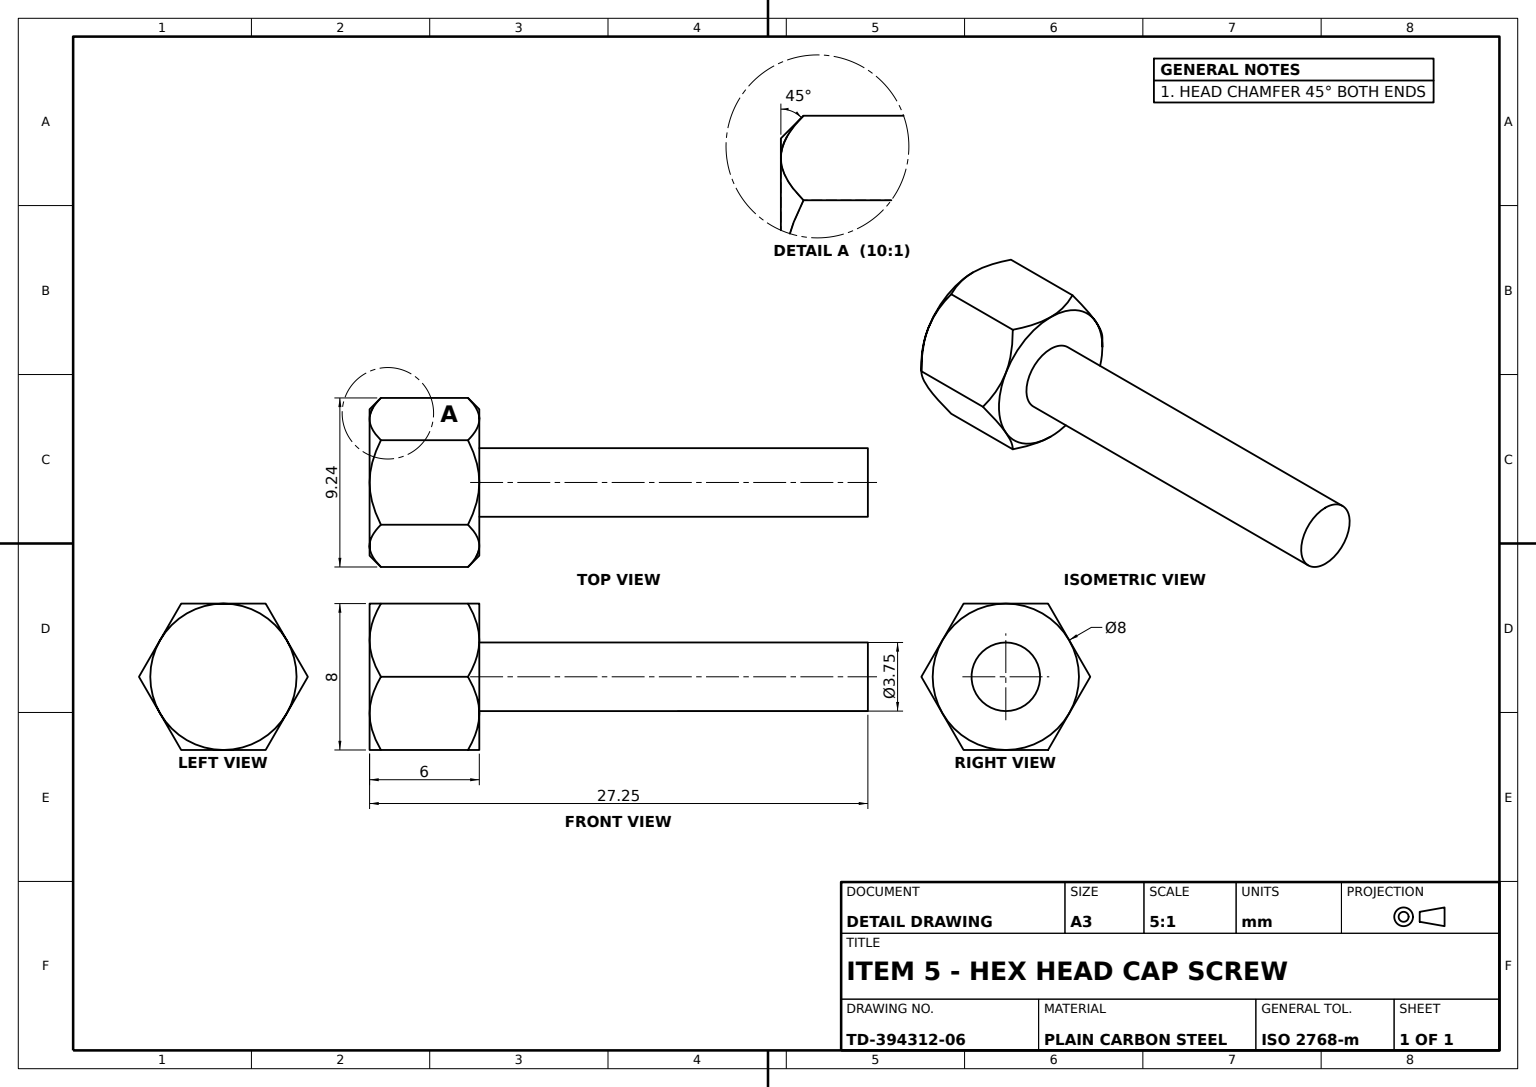
ISO-10303-21;
HEADER;
FILE_DESCRIPTION((''),'2;1');
FILE_NAME('','',(''),(''),'','','');
FILE_SCHEMA(('AUTOMOTIVE_DESIGN'));
ENDSEC;
DATA;
#1=APPLICATION_CONTEXT('');
#2=PRODUCT_CONTEXT('',#1,'mechanical');
#3=PRODUCT('','','',(#2));
#4=PRODUCT_DEFINITION_FORMATION('','',#3);
#5=PRODUCT_DEFINITION_CONTEXT('',#1,'design');
#6=PRODUCT_DEFINITION('','',#4,#5);
#7=PRODUCT_DEFINITION_SHAPE('','',#6);
#8=(LENGTH_UNIT()NAMED_UNIT(*)SI_UNIT(.MILLI.,.METRE.));
#9=(NAMED_UNIT(*)PLANE_ANGLE_UNIT()SI_UNIT($,.RADIAN.));
#10=(NAMED_UNIT(*)SI_UNIT($,.STERADIAN.)SOLID_ANGLE_UNIT());
#11=UNCERTAINTY_MEASURE_WITH_UNIT(LENGTH_MEASURE(1.E-05),#8,'distance_accuracy_value','');
#12=(GEOMETRIC_REPRESENTATION_CONTEXT(3)GLOBAL_UNCERTAINTY_ASSIGNED_CONTEXT((#11))GLOBAL_UNIT_ASSIGNED_CONTEXT((#8,#9,#10))REPRESENTATION_CONTEXT('',''));
#13=CARTESIAN_POINT('',(-2.309401,5.381198,4.));
#14=VERTEX_POINT('',#13);
#15=CARTESIAN_POINT('',(-2.309401,0.618802,4.));
#16=VERTEX_POINT('',#15);
#17=CARTESIAN_POINT('',(-2.309401,6.,4.));
#18=DIRECTION('',(0.,-1.,0.));
#19=VECTOR('',#18,1000.);
#20=LINE('',#17,#19);
#21=EDGE_CURVE('',#14,#16,#20,.T.);
#22=ORIENTED_EDGE('',*,*,#21,.F.);
#23=CARTESIAN_POINT('',(-3.464102,6.,2.));
#24=VERTEX_POINT('',#23);
#25=CARTESIAN_POINT('',(-3.263253,6.,2.34788));
#26=CARTESIAN_POINT('',(-3.065819,5.938579,2.689845));
#27=CARTESIAN_POINT('',(-2.67643,5.717205,3.364287));
#28=CARTESIAN_POINT('',(-2.490265,5.562062,3.686735));
#29=B_SPLINE_CURVE_WITH_KNOTS('',3,(#23,#25,#26,#27,#28,#13),.UNSPECIFIED.,.F.,.F.,(4,2,4),(0.002394158,0.003582724,0.00477129),.UNSPECIFIED.);
#30=EDGE_CURVE('',#24,#14,#29,.T.);
#31=ORIENTED_EDGE('',*,*,#30,.F.);
#32=CARTESIAN_POINT('',(-4.618802,5.381198,0.));
#33=VERTEX_POINT('',#32);
#34=CARTESIAN_POINT('',(-4.437729,5.562271,0.313628));
#35=CARTESIAN_POINT('',(-4.252558,5.716136,0.634354));
#36=CARTESIAN_POINT('',(-3.964816,5.880647,1.132738));
#37=CARTESIAN_POINT('',(-3.86722,5.924319,1.301778));
#38=CARTESIAN_POINT('',(-3.667881,5.984124,1.647044));
#39=CARTESIAN_POINT('',(-3.565234,6.,1.824833));
#40=B_SPLINE_CURVE_WITH_KNOTS('',3,(#32,#34,#35,#36,#37,#38,#39,#23),.UNSPECIFIED.,.F.,.F.,(4,2,2,4),(0.000000254,0.001197206,0.001795682,0.002394158),.UNSPECIFIED.);
#41=EDGE_CURVE('',#33,#24,#40,.T.);
#42=ORIENTED_EDGE('',*,*,#41,.F.);
#43=CARTESIAN_POINT('',(-4.618802,0.618802,0.));
#44=VERTEX_POINT('',#43);
#45=CARTESIAN_POINT('',(-4.618802,6.,0.));
#46=LINE('',#45,#19);
#47=EDGE_CURVE('',#33,#44,#46,.T.);
#48=ORIENTED_EDGE('',*,*,#47,.T.);
#49=CARTESIAN_POINT('',(-3.464102,0.,2.));
#50=VERTEX_POINT('',#49);
#51=CARTESIAN_POINT('',(-3.66495,0.,1.65212));
#52=CARTESIAN_POINT('',(-3.862384,0.061421,1.310155));
#53=CARTESIAN_POINT('',(-4.251773,0.282795,0.635713));
#54=CARTESIAN_POINT('',(-4.437938,0.437938,0.313265));
#55=B_SPLINE_CURVE_WITH_KNOTS('',3,(#49,#51,#52,#53,#54,#43),.UNSPECIFIED.,.F.,.F.,(4,2,4),(0.002394158,0.003582724,0.00477129),.UNSPECIFIED.);
#56=EDGE_CURVE('',#50,#44,#55,.T.);
#57=ORIENTED_EDGE('',*,*,#56,.F.);
#58=CARTESIAN_POINT('',(-2.490474,0.437729,3.686372));
#59=CARTESIAN_POINT('',(-2.675646,0.283864,3.365646));
#60=CARTESIAN_POINT('',(-2.963387,0.119353,2.867262));
#61=CARTESIAN_POINT('',(-3.060983,0.075681,2.698222));
#62=CARTESIAN_POINT('',(-3.260323,0.015876,2.352956));
#63=CARTESIAN_POINT('',(-3.362969,0.,2.175167));
#64=B_SPLINE_CURVE_WITH_KNOTS('',3,(#15,#58,#59,#60,#61,#62,#63,#49),.UNSPECIFIED.,.F.,.F.,(4,2,2,4),(0.000000254,0.001197206,0.001795682,0.002394158),.UNSPECIFIED.);
#65=EDGE_CURVE('',#16,#50,#64,.T.);
#66=ORIENTED_EDGE('',*,*,#65,.F.);
#67=EDGE_LOOP('',(#22,#31,#42,#48,#57,#66));
#68=FACE_OUTER_BOUND('',#67,.T.);
#69=DIRECTION('',(0.866025404,0.,-0.5));
#70=DIRECTION('',(-0.5,0.,-0.866025404));
#71=AXIS2_PLACEMENT_3D('',#45,#69,#70);
#72=PLANE('',#71);
#73=ADVANCED_FACE('',(#68),#72,.F.);
#74=CARTESIAN_POINT('',(2.309401,5.381198,4.));
#75=VERTEX_POINT('',#74);
#76=CARTESIAN_POINT('',(3.464102,6.,2.));
#77=VERTEX_POINT('',#76);
#78=CARTESIAN_POINT('',(2.490474,5.562271,3.686372));
#79=CARTESIAN_POINT('',(2.675646,5.716136,3.365646));
#80=CARTESIAN_POINT('',(2.963387,5.880647,2.867262));
#81=CARTESIAN_POINT('',(3.060983,5.924319,2.698222));
#82=CARTESIAN_POINT('',(3.260323,5.984124,2.352956));
#83=CARTESIAN_POINT('',(3.362969,6.,2.175167));
#84=B_SPLINE_CURVE_WITH_KNOTS('',3,(#74,#78,#79,#80,#81,#82,#83,#76),.UNSPECIFIED.,.F.,.F.,(4,2,2,4),(0.000000254,0.001197206,0.001795682,0.002394158),.UNSPECIFIED.);
#85=EDGE_CURVE('',#75,#77,#84,.T.);
#86=ORIENTED_EDGE('',*,*,#85,.T.);
#87=CARTESIAN_POINT('',(0.,6.,4.));
#88=VERTEX_POINT('',#87);
#89=CARTESIAN_POINT('',(0.,6.,0.));
#90=DIRECTION('',(0.,1.,0.));
#91=DIRECTION('',(0.,0.,1.));
#92=AXIS2_PLACEMENT_3D('',#89,#90,#91);
#93=CIRCLE('',#92,4.);
#94=EDGE_CURVE('',#88,#77,#93,.T.);
#95=ORIENTED_EDGE('',*,*,#94,.F.);
#96=CARTESIAN_POINT('',(0.406277,6.,4.));
#97=CARTESIAN_POINT('',(0.803107,5.937088,4.));
#98=CARTESIAN_POINT('',(1.383908,5.771434,4.));
#99=CARTESIAN_POINT('',(1.576064,5.704089,4.));
#100=CARTESIAN_POINT('',(1.949047,5.553691,4.));
#101=CARTESIAN_POINT('',(2.130932,5.470433,4.));
#102=B_SPLINE_CURVE_WITH_KNOTS('',3,(#87,#96,#97,#98,#99,#100,#101,#74),.UNSPECIFIED.,.F.,.F.,(4,2,2,4),(0.012126845,0.013335171,0.013939334,0.014543496),.UNSPECIFIED.);
#103=EDGE_CURVE('',#88,#75,#102,.T.);
#104=ORIENTED_EDGE('',*,*,#103,.T.);
#105=EDGE_LOOP('',(#86,#95,#104));
#106=FACE_OUTER_BOUND('',#105,.T.);
#107=AXIS2_PLACEMENT_3D('',#89,#18,#91);
#108=CONICAL_SURFACE('',#107,4.,0.785398163);
#109=ADVANCED_FACE('',(#106),#108,.T.);
#110=CARTESIAN_POINT('',(0.,-21.25,-1.875));
#111=VERTEX_POINT('',#110);
#112=CARTESIAN_POINT('',(0.,0.,-1.875));
#113=VERTEX_POINT('',#112);
#114=VECTOR('',#90,1000.);
#115=LINE('',#110,#114);
#116=EDGE_CURVE('',#111,#113,#115,.T.);
#117=ORIENTED_EDGE('',*,*,#116,.F.);
#118=CARTESIAN_POINT('',(0.,-21.25,1.875));
#119=VERTEX_POINT('',#118);
#120=CARTESIAN_POINT('',(0.,-21.25,0.));
#121=DIRECTION('',(0.,0.,-1.));
#122=AXIS2_PLACEMENT_3D('',#120,#18,#121);
#123=CIRCLE('',#122,1.875);
#124=EDGE_CURVE('',#119,#111,#123,.T.);
#125=ORIENTED_EDGE('',*,*,#124,.F.);
#126=CARTESIAN_POINT('',(0.,0.,1.875));
#127=VERTEX_POINT('',#126);
#128=LINE('',#118,#114);
#129=EDGE_CURVE('',#119,#127,#128,.T.);
#130=ORIENTED_EDGE('',*,*,#129,.T.);
#131=CARTESIAN_POINT('',(0.,0.,0.));
#132=AXIS2_PLACEMENT_3D('',#131,#18,#121);
#133=CIRCLE('',#132,1.875);
#134=EDGE_CURVE('',#127,#113,#133,.T.);
#135=ORIENTED_EDGE('',*,*,#134,.T.);
#136=EDGE_LOOP('',(#117,#125,#130,#135));
#137=FACE_OUTER_BOUND('',#136,.T.);
#138=AXIS2_PLACEMENT_3D('',#120,#90,#91);
#139=CYLINDRICAL_SURFACE('',#138,1.875);
#140=ADVANCED_FACE('',(#137),#139,.T.);
#141=CARTESIAN_POINT('',(2.309401,5.381198,-4.));
#142=VERTEX_POINT('',#141);
#143=CARTESIAN_POINT('',(2.309401,0.618802,-4.));
#144=VERTEX_POINT('',#143);
#145=CARTESIAN_POINT('',(2.309401,6.,-4.));
#146=LINE('',#145,#19);
#147=EDGE_CURVE('',#142,#144,#146,.T.);
#148=ORIENTED_EDGE('',*,*,#147,.T.);
#149=CARTESIAN_POINT('',(0.,0.,-4.));
#150=VERTEX_POINT('',#149);
#151=CARTESIAN_POINT('',(0.406277,0.,-4.));
#152=CARTESIAN_POINT('',(0.803107,0.062912,-4.));
#153=CARTESIAN_POINT('',(1.383908,0.228566,-4.));
#154=CARTESIAN_POINT('',(1.576064,0.295911,-4.));
#155=CARTESIAN_POINT('',(1.949047,0.446309,-4.));
#156=CARTESIAN_POINT('',(2.130932,0.529567,-4.));
#157=B_SPLINE_CURVE_WITH_KNOTS('',3,(#149,#151,#152,#153,#154,#155,#156,#143),.UNSPECIFIED.,.F.,.F.,(4,2,2,4),(0.012126845,0.013335171,0.013939334,0.014543496),.UNSPECIFIED.);
#158=EDGE_CURVE('',#150,#144,#157,.T.);
#159=ORIENTED_EDGE('',*,*,#158,.F.);
#160=CARTESIAN_POINT('',(-2.309401,0.618802,-4.));
#161=VERTEX_POINT('',#160);
#162=CARTESIAN_POINT('',(-2.12979,0.528996,-4.));
#163=CARTESIAN_POINT('',(-1.94713,0.445459,-4.));
#164=CARTESIAN_POINT('',(-1.57371,0.295039,-4.));
#165=CARTESIAN_POINT('',(-1.381886,0.227903,-4.));
#166=CARTESIAN_POINT('',(-0.801056,0.062501,-4.));
#167=CARTESIAN_POINT('',(-0.405791,0.,-4.));
#168=B_SPLINE_CURVE_WITH_KNOTS('',3,(#160,#162,#163,#164,#165,#166,#167,#149),.UNSPECIFIED.,.F.,.F.,(4,2,2,4),(0.009713081,0.010316522,0.010919963,0.012126845),.UNSPECIFIED.);
#169=EDGE_CURVE('',#161,#150,#168,.T.);
#170=ORIENTED_EDGE('',*,*,#169,.F.);
#171=CARTESIAN_POINT('',(-2.309401,5.381198,-4.));
#172=VERTEX_POINT('',#171);
#173=CARTESIAN_POINT('',(-2.309401,6.,-4.));
#174=LINE('',#173,#19);
#175=EDGE_CURVE('',#172,#161,#174,.T.);
#176=ORIENTED_EDGE('',*,*,#175,.F.);
#177=CARTESIAN_POINT('',(0.,6.,-4.));
#178=VERTEX_POINT('',#177);
#179=CARTESIAN_POINT('',(-0.406277,6.,-4.));
#180=CARTESIAN_POINT('',(-0.803107,5.937088,-4.));
#181=CARTESIAN_POINT('',(-1.383908,5.771434,-4.));
#182=CARTESIAN_POINT('',(-1.576064,5.704089,-4.));
#183=CARTESIAN_POINT('',(-1.949047,5.553691,-4.));
#184=CARTESIAN_POINT('',(-2.130932,5.470433,-4.));
#185=B_SPLINE_CURVE_WITH_KNOTS('',3,(#177,#179,#180,#181,#182,#183,#184,#171),.UNSPECIFIED.,.F.,.F.,(4,2,2,4),(0.012126845,0.013335171,0.013939334,0.014543496),.UNSPECIFIED.);
#186=EDGE_CURVE('',#178,#172,#185,.T.);
#187=ORIENTED_EDGE('',*,*,#186,.F.);
#188=CARTESIAN_POINT('',(2.12979,5.471004,-4.));
#189=CARTESIAN_POINT('',(1.94713,5.554541,-4.));
#190=CARTESIAN_POINT('',(1.57371,5.704961,-4.));
#191=CARTESIAN_POINT('',(1.381886,5.772097,-4.));
#192=CARTESIAN_POINT('',(0.801056,5.937499,-4.));
#193=CARTESIAN_POINT('',(0.405791,6.,-4.));
#194=B_SPLINE_CURVE_WITH_KNOTS('',3,(#141,#188,#189,#190,#191,#192,#193,#177),.UNSPECIFIED.,.F.,.F.,(4,2,2,4),(0.009713081,0.010316522,0.010919963,0.012126845),.UNSPECIFIED.);
#195=EDGE_CURVE('',#142,#178,#194,.T.);
#196=ORIENTED_EDGE('',*,*,#195,.F.);
#197=EDGE_LOOP('',(#148,#159,#170,#176,#187,#196));
#198=FACE_OUTER_BOUND('',#197,.T.);
#199=DIRECTION('',(1.,0.,0.));
#200=AXIS2_PLACEMENT_3D('',#145,#91,#199);
#201=PLANE('',#200);
#202=ADVANCED_FACE('',(#198),#201,.F.);
#203=CARTESIAN_POINT('',(2.309401,0.618802,4.));
#204=VERTEX_POINT('',#203);
#205=CARTESIAN_POINT('',(2.309401,6.,4.));
#206=LINE('',#205,#19);
#207=EDGE_CURVE('',#75,#204,#206,.T.);
#208=ORIENTED_EDGE('',*,*,#207,.F.);
#209=ORIENTED_EDGE('',*,*,#103,.F.);
#210=CARTESIAN_POINT('',(-2.12979,5.471004,4.));
#211=CARTESIAN_POINT('',(-1.94713,5.554541,4.));
#212=CARTESIAN_POINT('',(-1.57371,5.704961,4.));
#213=CARTESIAN_POINT('',(-1.381886,5.772097,4.));
#214=CARTESIAN_POINT('',(-0.801056,5.937499,4.));
#215=CARTESIAN_POINT('',(-0.405791,6.,4.));
#216=B_SPLINE_CURVE_WITH_KNOTS('',3,(#13,#210,#211,#212,#213,#214,#215,#87),.UNSPECIFIED.,.F.,.F.,(4,2,2,4),(0.009713081,0.010316522,0.010919963,0.012126845),.UNSPECIFIED.);
#217=EDGE_CURVE('',#14,#88,#216,.T.);
#218=ORIENTED_EDGE('',*,*,#217,.F.);
#219=ORIENTED_EDGE('',*,*,#21,.T.);
#220=CARTESIAN_POINT('',(0.,0.,4.));
#221=VERTEX_POINT('',#220);
#222=CARTESIAN_POINT('',(-0.406277,0.,4.));
#223=CARTESIAN_POINT('',(-0.803107,0.062912,4.));
#224=CARTESIAN_POINT('',(-1.383908,0.228566,4.));
#225=CARTESIAN_POINT('',(-1.576064,0.295911,4.));
#226=CARTESIAN_POINT('',(-1.949047,0.446309,4.));
#227=CARTESIAN_POINT('',(-2.130932,0.529567,4.));
#228=B_SPLINE_CURVE_WITH_KNOTS('',3,(#220,#222,#223,#224,#225,#226,#227,#15),.UNSPECIFIED.,.F.,.F.,(4,2,2,4),(0.012126845,0.013335171,0.013939334,0.014543496),.UNSPECIFIED.);
#229=EDGE_CURVE('',#221,#16,#228,.T.);
#230=ORIENTED_EDGE('',*,*,#229,.F.);
#231=CARTESIAN_POINT('',(2.12979,0.528996,4.));
#232=CARTESIAN_POINT('',(1.94713,0.445459,4.));
#233=CARTESIAN_POINT('',(1.57371,0.295039,4.));
#234=CARTESIAN_POINT('',(1.381886,0.227903,4.));
#235=CARTESIAN_POINT('',(0.801056,0.062501,4.));
#236=CARTESIAN_POINT('',(0.405791,0.,4.));
#237=B_SPLINE_CURVE_WITH_KNOTS('',3,(#203,#231,#232,#233,#234,#235,#236,#220),.UNSPECIFIED.,.F.,.F.,(4,2,2,4),(0.009713081,0.010316522,0.010919963,0.012126845),.UNSPECIFIED.);
#238=EDGE_CURVE('',#204,#221,#237,.T.);
#239=ORIENTED_EDGE('',*,*,#238,.F.);
#240=EDGE_LOOP('',(#208,#209,#218,#219,#230,#239));
#241=FACE_OUTER_BOUND('',#240,.T.);
#242=DIRECTION('',(-1.,0.,0.));
#243=AXIS2_PLACEMENT_3D('',#17,#121,#242);
#244=PLANE('',#243);
#245=ADVANCED_FACE('',(#241),#244,.F.);
#246=CARTESIAN_POINT('',(-3.464102,0.,-2.));
#247=VERTEX_POINT('',#246);
#248=CARTESIAN_POINT('',(-4.437729,0.437729,-0.313628));
#249=CARTESIAN_POINT('',(-4.252558,0.283864,-0.634354));
#250=CARTESIAN_POINT('',(-3.964816,0.119353,-1.132738));
#251=CARTESIAN_POINT('',(-3.86722,0.075681,-1.301778));
#252=CARTESIAN_POINT('',(-3.667881,0.015876,-1.647044));
#253=CARTESIAN_POINT('',(-3.565234,0.,-1.824833));
#254=B_SPLINE_CURVE_WITH_KNOTS('',3,(#43,#248,#249,#250,#251,#252,#253,#246),.UNSPECIFIED.,.F.,.F.,(4,2,2,4),(0.000000254,0.001197206,0.001795682,0.002394158),.UNSPECIFIED.);
#255=EDGE_CURVE('',#44,#247,#254,.T.);
#256=ORIENTED_EDGE('',*,*,#255,.T.);
#257=AXIS2_PLACEMENT_3D('',#131,#90,#91);
#258=CIRCLE('',#257,4.);
#259=EDGE_CURVE('',#247,#50,#258,.T.);
#260=ORIENTED_EDGE('',*,*,#259,.T.);
#261=ORIENTED_EDGE('',*,*,#56,.T.);
#262=EDGE_LOOP('',(#256,#260,#261));
#263=FACE_OUTER_BOUND('',#262,.T.);
#264=AXIS2_PLACEMENT_3D('',#131,#90,#121);
#265=CONICAL_SURFACE('',#264,4.,0.785398163);
#266=ADVANCED_FACE('',(#263),#265,.T.);
#267=EDGE_CURVE('',#111,#119,#123,.T.);
#268=ORIENTED_EDGE('',*,*,#267,.F.);
#269=ORIENTED_EDGE('',*,*,#116,.T.);
#270=EDGE_CURVE('',#113,#127,#133,.T.);
#271=ORIENTED_EDGE('',*,*,#270,.T.);
#272=ORIENTED_EDGE('',*,*,#129,.F.);
#273=EDGE_LOOP('',(#268,#269,#271,#272));
#274=FACE_OUTER_BOUND('',#273,.T.);
#275=ADVANCED_FACE('',(#274),#139,.T.);
#276=CARTESIAN_POINT('',(3.464102,0.,-2.));
#277=VERTEX_POINT('',#276);
#278=CARTESIAN_POINT('',(4.618802,0.618802,0.));
#279=VERTEX_POINT('',#278);
#280=CARTESIAN_POINT('',(3.66495,0.,-1.65212));
#281=CARTESIAN_POINT('',(3.862384,0.061421,-1.310155));
#282=CARTESIAN_POINT('',(4.251773,0.282795,-0.635713));
#283=CARTESIAN_POINT('',(4.437938,0.437938,-0.313265));
#284=B_SPLINE_CURVE_WITH_KNOTS('',3,(#276,#280,#281,#282,#283,#278),.UNSPECIFIED.,.F.,.F.,(4,2,4),(0.002394158,0.003582724,0.00477129),.UNSPECIFIED.);
#285=EDGE_CURVE('',#277,#279,#284,.T.);
#286=ORIENTED_EDGE('',*,*,#285,.T.);
#287=CARTESIAN_POINT('',(3.464102,0.,2.));
#288=VERTEX_POINT('',#287);
#289=CARTESIAN_POINT('',(4.437729,0.437729,0.313628));
#290=CARTESIAN_POINT('',(4.252558,0.283864,0.634354));
#291=CARTESIAN_POINT('',(3.964816,0.119353,1.132738));
#292=CARTESIAN_POINT('',(3.86722,0.075681,1.301778));
#293=CARTESIAN_POINT('',(3.667881,0.015876,1.647044));
#294=CARTESIAN_POINT('',(3.565234,0.,1.824833));
#295=B_SPLINE_CURVE_WITH_KNOTS('',3,(#278,#289,#290,#291,#292,#293,#294,#287),.UNSPECIFIED.,.F.,.F.,(4,2,2,4),(0.000000254,0.001197206,0.001795682,0.002394158),.UNSPECIFIED.);
#296=EDGE_CURVE('',#279,#288,#295,.T.);
#297=ORIENTED_EDGE('',*,*,#296,.T.);
#298=EDGE_CURVE('',#288,#277,#258,.T.);
#299=ORIENTED_EDGE('',*,*,#298,.T.);
#300=EDGE_LOOP('',(#286,#297,#299));
#301=FACE_OUTER_BOUND('',#300,.T.);
#302=ADVANCED_FACE('',(#301),#265,.T.);
#303=CARTESIAN_POINT('',(-3.263253,0.,-2.34788));
#304=CARTESIAN_POINT('',(-3.065819,0.061421,-2.689845));
#305=CARTESIAN_POINT('',(-2.67643,0.282795,-3.364287));
#306=CARTESIAN_POINT('',(-2.490265,0.437938,-3.686735));
#307=B_SPLINE_CURVE_WITH_KNOTS('',3,(#246,#303,#304,#305,#306,#160),.UNSPECIFIED.,.F.,.F.,(4,2,4),(0.002394158,0.003582724,0.00477129),.UNSPECIFIED.);
#308=EDGE_CURVE('',#247,#161,#307,.T.);
#309=ORIENTED_EDGE('',*,*,#308,.F.);
#310=ORIENTED_EDGE('',*,*,#255,.F.);
#311=ORIENTED_EDGE('',*,*,#47,.F.);
#312=CARTESIAN_POINT('',(-3.464102,6.,-2.));
#313=VERTEX_POINT('',#312);
#314=CARTESIAN_POINT('',(-3.66495,6.,-1.65212));
#315=CARTESIAN_POINT('',(-3.862384,5.938579,-1.310155));
#316=CARTESIAN_POINT('',(-4.251773,5.717205,-0.635713));
#317=CARTESIAN_POINT('',(-4.437938,5.562062,-0.313265));
#318=B_SPLINE_CURVE_WITH_KNOTS('',3,(#312,#314,#315,#316,#317,#32),.UNSPECIFIED.,.F.,.F.,(4,2,4),(0.002394158,0.003582724,0.00477129),.UNSPECIFIED.);
#319=EDGE_CURVE('',#313,#33,#318,.T.);
#320=ORIENTED_EDGE('',*,*,#319,.F.);
#321=CARTESIAN_POINT('',(-2.490474,5.562271,-3.686372));
#322=CARTESIAN_POINT('',(-2.675646,5.716136,-3.365646));
#323=CARTESIAN_POINT('',(-2.963387,5.880647,-2.867262));
#324=CARTESIAN_POINT('',(-3.060983,5.924319,-2.698222));
#325=CARTESIAN_POINT('',(-3.260323,5.984124,-2.352956));
#326=CARTESIAN_POINT('',(-3.362969,6.,-2.175167));
#327=B_SPLINE_CURVE_WITH_KNOTS('',3,(#171,#321,#322,#323,#324,#325,#326,#312),.UNSPECIFIED.,.F.,.F.,(4,2,2,4),(0.000000254,0.001197206,0.001795682,0.002394158),.UNSPECIFIED.);
#328=EDGE_CURVE('',#172,#313,#327,.T.);
#329=ORIENTED_EDGE('',*,*,#328,.F.);
#330=ORIENTED_EDGE('',*,*,#175,.T.);
#331=EDGE_LOOP('',(#309,#310,#311,#320,#329,#330));
#332=FACE_OUTER_BOUND('',#331,.T.);
#333=DIRECTION('',(0.866025404,0.,0.5));
#334=DIRECTION('',(0.5,0.,-0.866025404));
#335=AXIS2_PLACEMENT_3D('',#173,#333,#334);
#336=PLANE('',#335);
#337=ADVANCED_FACE('',(#332),#336,.F.);
#338=ORIENTED_EDGE('',*,*,#147,.F.);
#339=CARTESIAN_POINT('',(3.464102,6.,-2.));
#340=VERTEX_POINT('',#339);
#341=CARTESIAN_POINT('',(3.263253,6.,-2.34788));
#342=CARTESIAN_POINT('',(3.065819,5.938579,-2.689845));
#343=CARTESIAN_POINT('',(2.67643,5.717205,-3.364287));
#344=CARTESIAN_POINT('',(2.490265,5.562062,-3.686735));
#345=B_SPLINE_CURVE_WITH_KNOTS('',3,(#339,#341,#342,#343,#344,#141),.UNSPECIFIED.,.F.,.F.,(4,2,4),(0.002394158,0.003582724,0.00477129),.UNSPECIFIED.);
#346=EDGE_CURVE('',#340,#142,#345,.T.);
#347=ORIENTED_EDGE('',*,*,#346,.F.);
#348=CARTESIAN_POINT('',(4.618802,5.381198,0.));
#349=VERTEX_POINT('',#348);
#350=CARTESIAN_POINT('',(4.437729,5.562271,-0.313628));
#351=CARTESIAN_POINT('',(4.252558,5.716136,-0.634354));
#352=CARTESIAN_POINT('',(3.964816,5.880647,-1.132738));
#353=CARTESIAN_POINT('',(3.86722,5.924319,-1.301778));
#354=CARTESIAN_POINT('',(3.667881,5.984124,-1.647044));
#355=CARTESIAN_POINT('',(3.565234,6.,-1.824833));
#356=B_SPLINE_CURVE_WITH_KNOTS('',3,(#348,#350,#351,#352,#353,#354,#355,#339),.UNSPECIFIED.,.F.,.F.,(4,2,2,4),(0.000000254,0.001197206,0.001795682,0.002394158),.UNSPECIFIED.);
#357=EDGE_CURVE('',#349,#340,#356,.T.);
#358=ORIENTED_EDGE('',*,*,#357,.F.);
#359=CARTESIAN_POINT('',(4.618802,6.,0.));
#360=LINE('',#359,#19);
#361=EDGE_CURVE('',#349,#279,#360,.T.);
#362=ORIENTED_EDGE('',*,*,#361,.T.);
#363=ORIENTED_EDGE('',*,*,#285,.F.);
#364=CARTESIAN_POINT('',(2.490474,0.437729,-3.686372));
#365=CARTESIAN_POINT('',(2.675646,0.283864,-3.365646));
#366=CARTESIAN_POINT('',(2.963387,0.119353,-2.867262));
#367=CARTESIAN_POINT('',(3.060983,0.075681,-2.698222));
#368=CARTESIAN_POINT('',(3.260323,0.015876,-2.352956));
#369=CARTESIAN_POINT('',(3.362969,0.,-2.175167));
#370=B_SPLINE_CURVE_WITH_KNOTS('',3,(#143,#364,#365,#366,#367,#368,#369,#276),.UNSPECIFIED.,.F.,.F.,(4,2,2,4),(0.000000254,0.001197206,0.001795682,0.002394158),.UNSPECIFIED.);
#371=EDGE_CURVE('',#144,#277,#370,.T.);
#372=ORIENTED_EDGE('',*,*,#371,.F.);
#373=EDGE_LOOP('',(#338,#347,#358,#362,#363,#372));
#374=FACE_OUTER_BOUND('',#373,.T.);
#375=DIRECTION('',(-0.866025404,0.,0.5));
#376=DIRECTION('',(0.5,0.,0.866025404));
#377=AXIS2_PLACEMENT_3D('',#359,#375,#376);
#378=PLANE('',#377);
#379=ADVANCED_FACE('',(#374),#378,.F.);
#380=ORIENTED_EDGE('',*,*,#217,.T.);
#381=EDGE_CURVE('',#24,#88,#93,.T.);
#382=ORIENTED_EDGE('',*,*,#381,.F.);
#383=ORIENTED_EDGE('',*,*,#30,.T.);
#384=EDGE_LOOP('',(#380,#382,#383));
#385=FACE_OUTER_BOUND('',#384,.T.);
#386=ADVANCED_FACE('',(#385),#108,.T.);
#387=ORIENTED_EDGE('',*,*,#371,.T.);
#388=CIRCLE('',#132,4.);
#389=EDGE_CURVE('',#150,#277,#388,.T.);
#390=ORIENTED_EDGE('',*,*,#389,.F.);
#391=ORIENTED_EDGE('',*,*,#158,.T.);
#392=EDGE_LOOP('',(#387,#390,#391));
#393=FACE_OUTER_BOUND('',#392,.T.);
#394=ADVANCED_FACE('',(#393),#265,.T.);
#395=ORIENTED_EDGE('',*,*,#319,.T.);
#396=ORIENTED_EDGE('',*,*,#41,.T.);
#397=EDGE_CURVE('',#313,#24,#93,.T.);
#398=ORIENTED_EDGE('',*,*,#397,.F.);
#399=EDGE_LOOP('',(#395,#396,#398));
#400=FACE_OUTER_BOUND('',#399,.T.);
#401=ADVANCED_FACE('',(#400),#108,.T.);
#402=ORIENTED_EDGE('',*,*,#397,.T.);
#403=ORIENTED_EDGE('',*,*,#381,.T.);
#404=ORIENTED_EDGE('',*,*,#94,.T.);
#405=EDGE_CURVE('',#77,#340,#93,.T.);
#406=ORIENTED_EDGE('',*,*,#405,.T.);
#407=EDGE_CURVE('',#340,#178,#93,.T.);
#408=ORIENTED_EDGE('',*,*,#407,.T.);
#409=EDGE_CURVE('',#178,#313,#93,.T.);
#410=ORIENTED_EDGE('',*,*,#409,.T.);
#411=EDGE_LOOP('',(#402,#403,#404,#406,#408,#410));
#412=FACE_OUTER_BOUND('',#411,.T.);
#413=PLANE('',#92);
#414=ADVANCED_FACE('',(#412),#413,.T.);
#415=ORIENTED_EDGE('',*,*,#65,.T.);
#416=EDGE_CURVE('',#50,#221,#258,.T.);
#417=ORIENTED_EDGE('',*,*,#416,.T.);
#418=ORIENTED_EDGE('',*,*,#229,.T.);
#419=EDGE_LOOP('',(#415,#417,#418));
#420=FACE_OUTER_BOUND('',#419,.T.);
#421=ADVANCED_FACE('',(#420),#265,.T.);
#422=ORIENTED_EDGE('',*,*,#267,.T.);
#423=ORIENTED_EDGE('',*,*,#124,.T.);
#424=EDGE_LOOP('',(#422,#423));
#425=FACE_OUTER_BOUND('',#424,.T.);
#426=PLANE('',#122);
#427=ADVANCED_FACE('',(#425),#426,.T.);
#428=ORIENTED_EDGE('',*,*,#407,.F.);
#429=ORIENTED_EDGE('',*,*,#346,.T.);
#430=ORIENTED_EDGE('',*,*,#195,.T.);
#431=EDGE_LOOP('',(#428,#429,#430));
#432=FACE_OUTER_BOUND('',#431,.T.);
#433=ADVANCED_FACE('',(#432),#108,.T.);
#434=ORIENTED_EDGE('',*,*,#85,.F.);
#435=ORIENTED_EDGE('',*,*,#207,.T.);
#436=CARTESIAN_POINT('',(3.263253,0.,2.34788));
#437=CARTESIAN_POINT('',(3.065819,0.061421,2.689845));
#438=CARTESIAN_POINT('',(2.67643,0.282795,3.364287));
#439=CARTESIAN_POINT('',(2.490265,0.437938,3.686735));
#440=B_SPLINE_CURVE_WITH_KNOTS('',3,(#287,#436,#437,#438,#439,#203),.UNSPECIFIED.,.F.,.F.,(4,2,4),(0.002394158,0.003582724,0.00477129),.UNSPECIFIED.);
#441=EDGE_CURVE('',#288,#204,#440,.T.);
#442=ORIENTED_EDGE('',*,*,#441,.F.);
#443=ORIENTED_EDGE('',*,*,#296,.F.);
#444=ORIENTED_EDGE('',*,*,#361,.F.);
#445=CARTESIAN_POINT('',(3.66495,6.,1.65212));
#446=CARTESIAN_POINT('',(3.862384,5.938579,1.310155));
#447=CARTESIAN_POINT('',(4.251773,5.717205,0.635713));
#448=CARTESIAN_POINT('',(4.437938,5.562062,0.313265));
#449=B_SPLINE_CURVE_WITH_KNOTS('',3,(#76,#445,#446,#447,#448,#348),.UNSPECIFIED.,.F.,.F.,(4,2,4),(0.002394158,0.003582724,0.00477129),.UNSPECIFIED.);
#450=EDGE_CURVE('',#77,#349,#449,.T.);
#451=ORIENTED_EDGE('',*,*,#450,.F.);
#452=EDGE_LOOP('',(#434,#435,#442,#443,#444,#451));
#453=FACE_OUTER_BOUND('',#452,.T.);
#454=DIRECTION('',(-0.866025404,0.,-0.5));
#455=DIRECTION('',(-0.5,0.,0.866025404));
#456=AXIS2_PLACEMENT_3D('',#205,#454,#455);
#457=PLANE('',#456);
#458=ADVANCED_FACE('',(#453),#457,.F.);
#459=EDGE_CURVE('',#221,#288,#258,.T.);
#460=ORIENTED_EDGE('',*,*,#459,.F.);
#461=ORIENTED_EDGE('',*,*,#416,.F.);
#462=ORIENTED_EDGE('',*,*,#259,.F.);
#463=EDGE_CURVE('',#150,#247,#258,.T.);
#464=ORIENTED_EDGE('',*,*,#463,.F.);
#465=ORIENTED_EDGE('',*,*,#389,.T.);
#466=ORIENTED_EDGE('',*,*,#298,.F.);
#467=EDGE_LOOP('',(#460,#461,#462,#464,#465,#466));
#468=FACE_OUTER_BOUND('',#467,.T.);
#469=ORIENTED_EDGE('',*,*,#270,.F.);
#470=ORIENTED_EDGE('',*,*,#134,.F.);
#471=EDGE_LOOP('',(#469,#470));
#472=FACE_BOUND('',#471,.T.);
#473=PLANE('',#257);
#474=ADVANCED_FACE('',(#468,#472),#473,.F.);
#475=ORIENTED_EDGE('',*,*,#441,.T.);
#476=ORIENTED_EDGE('',*,*,#238,.T.);
#477=ORIENTED_EDGE('',*,*,#459,.T.);
#478=EDGE_LOOP('',(#475,#476,#477));
#479=FACE_OUTER_BOUND('',#478,.T.);
#480=ADVANCED_FACE('',(#479),#265,.T.);
#481=ORIENTED_EDGE('',*,*,#450,.T.);
#482=ORIENTED_EDGE('',*,*,#357,.T.);
#483=ORIENTED_EDGE('',*,*,#405,.F.);
#484=EDGE_LOOP('',(#481,#482,#483));
#485=FACE_OUTER_BOUND('',#484,.T.);
#486=ADVANCED_FACE('',(#485),#108,.T.);
#487=ORIENTED_EDGE('',*,*,#169,.T.);
#488=ORIENTED_EDGE('',*,*,#463,.T.);
#489=ORIENTED_EDGE('',*,*,#308,.T.);
#490=EDGE_LOOP('',(#487,#488,#489));
#491=FACE_OUTER_BOUND('',#490,.T.);
#492=ADVANCED_FACE('',(#491),#265,.T.);
#493=ORIENTED_EDGE('',*,*,#409,.F.);
#494=ORIENTED_EDGE('',*,*,#186,.T.);
#495=ORIENTED_EDGE('',*,*,#328,.T.);
#496=EDGE_LOOP('',(#493,#494,#495));
#497=FACE_OUTER_BOUND('',#496,.T.);
#498=ADVANCED_FACE('',(#497),#108,.T.);
#499=CLOSED_SHELL('',(#73,#109,#140,#202,#245,#266,#275,#302,#337,#379,#386,#394,#401,#414,#421,#427,#433,#458,#474,#480,#486,#492,#498));
#500=MANIFOLD_SOLID_BREP('',#499);
#501=ADVANCED_BREP_SHAPE_REPRESENTATION('',(#500),#12);
#502=SHAPE_DEFINITION_REPRESENTATION(#7,#501);
ENDSEC;
END-ISO-10303-21;
